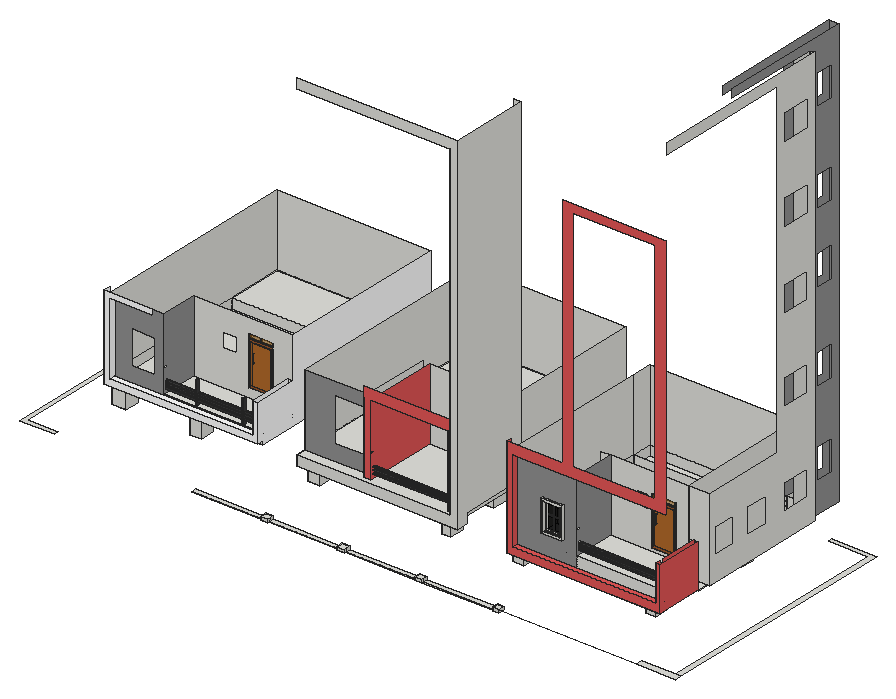
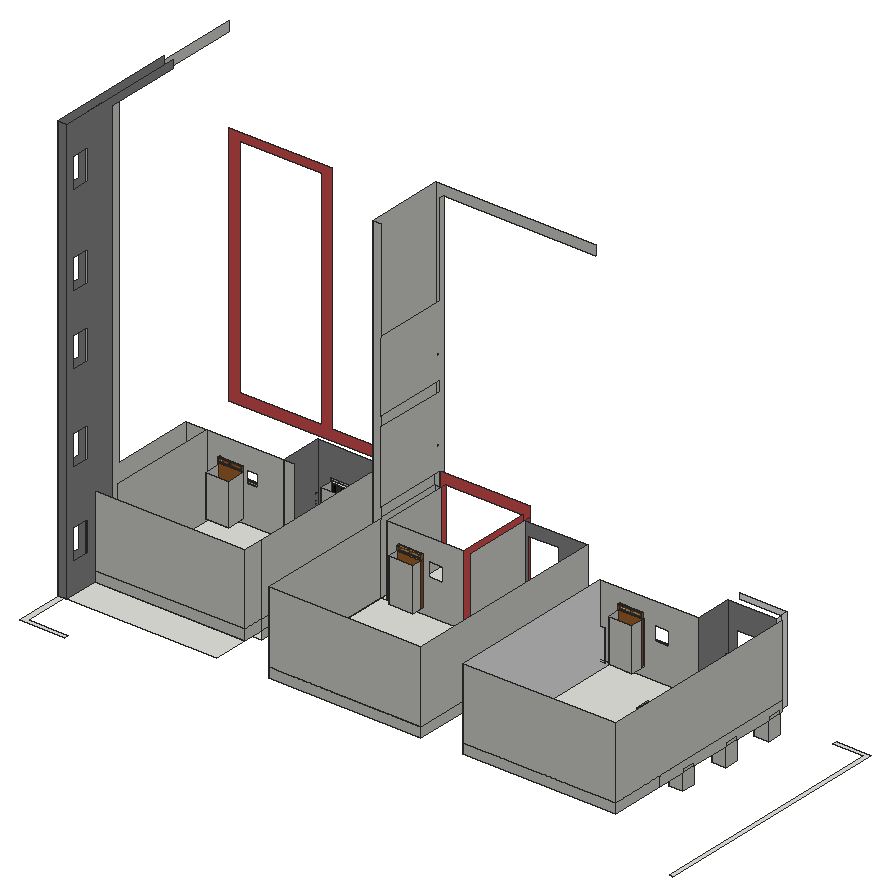
# SketchUp Ruby script. Lengths in inches.
U = 1.inch
M = Sketchup.active_model
def pt(a) = Geom::Point3d.new(a.map { |v| v * U })
def face(e, loops, mat)
  f = e.add_face(loops[0].map { |a| pt(a) })
  loops[1..].each { |l| e.add_face(l.map { |a| pt(a) }).erase! }
  f.material = f.back_material = mat if mat
  f
end
# faces: each face lists its corners as indices into pts; further lists are holes
def faces(e, pts, list, mat = nil) = list.each { |f| face(e, (f[0].is_a?(Array) ? f : [f]).map { |l| l.map { |i| pts[i] } }, mat) }
# xy, xz, yz: faces in a plane at the given z, y or x. An outline is a flat list of corners, or four numbers for a rectangle; further outlines are holes
def ring(l) = l.size == 4 ? [[l[0], l[1]], [l[2], l[1]], [l[2], l[3]], [l[0], l[3]]] : l.each_slice(2).to_a
def flat(e, list, mat, &to3) = list.each { |f| face(e, (f[0].is_a?(Array) ? f : [f]).map { |l| ring(l).map { |u, v| to3.(u, v) } }, mat) }
def xy(e, z, list, mat = nil) = flat(e, list, mat) { |x, y| [x, y, z] }
def xz(e, y, list, mat = nil) = flat(e, list, mat) { |x, z| [x, y, z] }
def yz(e, x, list, mat = nil) = flat(e, list, mat) { |y, z| [x, y, z] }
def lines(e, pts, list) = list.each { |a, b| e.add_line(pt(pts[a]), pt(pts[b])) }
# prism: a flat outline (further loops are holes) pulled along v
def prism(e, loops, v, mat = nil)
  f = face(e, loops, mat); d = Geom::Vector3d.new(v.map { |x| x * U })
  f.pushpull(f.normal.samedirection?(d) ? d.length : -d.length)
end
def box(e, o, s, mat = nil) = prism(e, [[o, [o[0] + s[0], o[1], o[2]], [o[0] + s[0], o[1] + s[1], o[2]], [o[0], o[1] + s[1], o[2]]]], [0, 0, s[2]], mat)
def at(x, y, z, deg = 0) = Geom::Transformation.translation(pt([x, y, z])) * Geom::Transformation.rotation(ORIGIN, Z_AXIS, deg.degrees)
def axes(o, x, y, z) = Geom::Transformation.new([*x, 0, *y, 0, *z, 0, *pt(o).to_a, 1])
def part(name) = M.definitions.add(name)
# library, detail: a bought-in or finely detailed component or shape, given as its bounding box
def library(name, o, s) = part(name).tap { |d| box(d.entities, o, s) }
def detail(e, o, s) = box(e.add_group.entities, o, s)
def put(e, d, t, mat = nil) = e.add_instance(d, t).tap { |i| i.material = mat if mat }
def group(e, t, mat = nil) = e.add_group.tap { |g| g.transformation = t; g.material = mat if mat }.entities
root = M.entities
M.materials.add("Generic").color = [145, 145, 145]
M.materials.add("Generic\#2").color = [229, 87, 87]
M.materials.add("[Color M00]").color = [255, 255, 255]
M.materials.add("[Color M07]").color = [58, 58, 58]
M.materials.add("[Color M08]").color = [45, 45, 45]
M.materials.add("[Translucent Glass Dark Green]").color = [168, 100, 12]
M.materials["[Translucent Glass Dark Green]"].alpha = 0.5
M.materials.add("[Translucent Glass Gray]").color = [0, 0, 0]
M.materials["[Translucent Glass Gray]"].alpha = 0.62
M.materials.add("[Wood Bamboo]").color = [177, 105, 43]
M.materials.add("[Wood Cherry Original]").color = [152, 86, 42]
c1 = part("Group\#10")
xy(c1.entities,0,[[0,1.08,55.8125,6.01]],"[Wood Cherry Original]")
xy(c1.entities,3.96,[[3.96,1.08,51.86,3.01]],"[Wood Bamboo]")
xy(c1.entities,51.66,[[8.63,0,9.88,3.01]],"[Color M08]")
xy(c1.entities,52.54,[[8.63,0.6875,9.88,3.01]],"[Color M08]")
xy(c1.entities,71.82,[[8.63,0.6875,9.88,3.01]],"[Color M08]")
xy(c1.entities,72.69,[[8.63,0,9.88,3.01]],"[Color M08]")
xy(c1.entities,97.36,[[3.96,1.08,51.86,3.01]],"[Wood Bamboo]")
xy(c1.entities,101.3125,[[0,1.08,55.8125,6.01]],"[Wood Bamboo]")
xy(c1.entities,102.55,[[1.23,1.08,27.29,3.01],[27.29,1.08,28.52,1.95],[28.52,1.08,54.58,3.01]],"[Wood Bamboo]")
xy(c1.entities,112.31,[[1.23,1.08,1.23,3.01,27.29,3.01,27.29,1.95,28.52,1.95,28.52,3.01,54.58,3.01,54.58,1.08]],"[Wood Bamboo]")
xy(c1.entities,113.54,[[0,1.08,55.8125,6.01]],"[Wood Bamboo]")
xz(c1.entities,0,[[8.63,51.66,9.88,72.69]],"[Color M08]")
xz(c1.entities,0.6875,[[8.63,52.54,9.88,71.82]])
xz(c1.entities,1.08,[[0,101.3125,55.8125,102.55],[0,102.55,1.23,102.55,1.23,112.31,54.58,112.31,54.58,102.55,55.8125,102.55,55.8125,113.54,0,113.54]],"[Wood Bamboo]")
xz(c1.entities,1.08,[[[0,0,55.8125,101.3125],[3.96,3.96,51.86,97.36]]],"[Wood Cherry Original]")
xz(c1.entities,1.95,[[27.29,102.55,28.52,112.31]],"[Wood Bamboo]")
xz(c1.entities,3.01,[[8.63,71.82,9.88,72.69]])
xz(c1.entities,3.01,[[1.23,102.55,27.29,112.31],[28.52,102.55,54.58,112.31]],"[Translucent Glass Dark Green]")
xz(c1.entities,3.01,[[[3.96,3.96,51.86,97.36],[8.63,71.82,9.88,72.69],[8.63,51.66,9.88,52.54]]],"[Wood Bamboo]")
xz(c1.entities,6.01,[[0,0,55.8125,101.3125],[0,112.31,55.8125,113.54]],"[Wood Bamboo]")
yz(c1.entities,0,[[1.08,101.3125,6.01,113.54]],"[Wood Bamboo]")
yz(c1.entities,0,[[1.08,0,6.01,101.3125]],"[Wood Cherry Original]")
yz(c1.entities,1.23,[[1.08,102.55,3.01,112.31]],"[Wood Bamboo]")
yz(c1.entities,3.96,[[1.08,3.96,3.01,97.36]],"[Wood Bamboo]")
yz(c1.entities,8.63,[[0,51.66,0,72.69,3.01,72.69,3.01,71.82,0.6875,71.82,0.6875,52.54,3.01,52.54,3.01,51.66]],"[Color M08]")
yz(c1.entities,9.88,[[0,51.66,3.01,51.66,3.01,52.54,0.6875,52.54,0.6875,71.82,3.01,71.82,3.01,72.69,0,72.69]],"[Color M08]")
yz(c1.entities,27.29,[[1.95,102.55,3.01,112.31]],"[Wood Bamboo]")
yz(c1.entities,28.52,[[1.95,102.55,3.01,112.31]],"[Wood Bamboo]")
yz(c1.entities,51.86,[[1.08,3.96,3.01,97.36]],"[Wood Bamboo]")
yz(c1.entities,54.58,[[1.08,102.55,3.01,112.31]],"[Wood Bamboo]")
yz(c1.entities,55.8125,[[1.08,101.3125,6.01,113.54]],"[Wood Bamboo]")
yz(c1.entities,55.8125,[[1.08,0,6.01,101.3125]],"[Wood Cherry Original]")
p = [[1.23,3.01,112.31],[1.23,6.01,112.31],[9.24,3.01,71.99],[9.24,0.51,71.99],[9.24,0.51,52.37],[9.24,3.01,52.37]]
lines(c1.entities,p,[[0,1],[2,3],[3,4],[4,5]])
c2 = part("Group\#1")
xy(c2.entities,0,[[0,0,39.9375,6]])
xy(c2.entities,3.79,[[3.79,0,36.15,3]])
xy(c2.entities,60.83,[[3.79,0,36.15,3]])
xy(c2.entities,64.62,[[0,0,39.9375,6]])
xz(c2.entities,0,[[[0,0,39.9375,64.62],[3.79,3.79,36.15,60.83]]])
xz(c2.entities,3,[[18.07,3.79,20.49,3.79,20.49,32.1,36.15,32.1,36.15,34.21,20.49,34.21,20.49,60.83,18.07,60.83,18.07,34.21,3.79,34.21,3.79,32.1,18.07,32.1]],"[Color M08]")
xz(c2.entities,3,[[3.79,3.79,18.07,32.1],[20.49,3.79,36.15,32.1],[3.79,34.21,18.07,60.83],[20.49,34.21,36.15,60.83]],"[Translucent Glass Gray]")
xz(c2.entities,6,[[0,0,39.9375,64.62]],"[Translucent Glass Gray]")
yz(c2.entities,0,[[0,0,6,64.62]])
yz(c2.entities,3.79,[[0,3.79,3,60.83]])
yz(c2.entities,36.15,[[0,3.79,3,60.83]])
yz(c2.entities,39.9375,[[0,0,6,64.62]])
box(root,[317.97,107.54,123.46],[28.18,32.5,52.04])
box(root,[317.97,359.61,128.98],[28.18,32.5,46.52])
box(root,[317.97,233.58,128.98],[28.18,32.5,46.52])
xy(root,77.4375,[[566.41,4.0625,583.85,19.0625],[746.02,4.0625,763.9,19.0625],[927.64,4.0625,943.95,19.0625],[1109.75,4.0625,1124,19.0625],[403.8,5.5,566.41,8.375],
  [583.85,5.5,746.02,8.375],[763.9,5.5,927.64,8.375],[943.95,5.5,1109.75,8.375],[403.8,8.375,566.41,19.0625],[583.85,8.375,746.02,19.0625],
  [763.9,8.375,927.64,19.0625],[943.95,8.375,1109.75,19.0625]])
xy(root,84,[[566.41,4.0625,583.85,19.0625],[746.02,4.0625,763.9,19.0625],[927.64,4.0625,943.95,19.0625],[1109.75,4.0625,1124,19.0625],[1447.36,4.0625,1540.27,19.0625],
  [0,8.375,80.43,8.375,80.43,19.0625,8.1875,19.0625,8.1875,590.625,0,590.625],[1528.71,19.0625,1540.27,19.0625,1540.27,590.625,1435.83,590.625,1435.83,580.6875,1528.71,580.6875]])
xy(root,117.37,[[1385.5,359.61,1409.07,392.11]])
xy(root,123.46,[[135.5,107.54,168.88,107.54,135.5,140.04],[168.88,107.54,168.88,140.04,135.5,140.04],[594.11,107.54,622.68,140.04],[909.52,107.54,930.58,140.04],[1075.83,107.54,1100.54,140.04],
  [1385.5,107.54,1409.07,140.04],[135.5,233.58,168.88,266.08],[1385.5,233.58,1409.07,266.08]])
xy(root,128.98,[[909.52,233.58,930.58,266.08],[135.5,359.61,168.88,392.11],[909.52,359.61,930.58,392.11],[1075.83,359.61,1100.54,392.11]])
xy(root,132.52,[[594.11,359.61,622.68,392.11]])
xy(root,148.75,[[1075.83,88,1435.83,99.8125],[[1075.83,99.8125,1075.83,107.54,1100.54,107.54,1100.54,140.04,1075.83,140.04,1075.83,233.58,1100.54,233.58,1100.54,266.08,1075.83,266.08,1075.83,359.61,1100.54,359.61,1100.54,392.11,1075.83,392.11,1075.83,459.8125,1435.83,459.8125,1435.83,99.8125],[1385.5,359.61,1409.07,392.11],[1385.5,233.58,1409.07,266.08],[1385.5,107.54,1409.07,140.04]],[1075.83,107.54,1100.54,140.04],[1075.83,233.58,1100.54,266.08],[1075.83,359.61,1100.54,392.11]])
xy(root,168,[[[594.11,74.75,594.11,107.54,622.68,107.54,622.68,140.04,594.11,140.04,594.11,233.58,622.68,233.58,622.68,266.08,594.11,266.08,594.11,359.61,622.68,359.61,622.68,392.11,594.11,392.11,594.11,459.8125,954.11,459.8125,954.11,99.8125,972.24,99.8125,972.24,74.75],[909.52,359.61,930.58,392.11],[909.52,233.58,930.58,266.08],[909.52,107.54,930.58,140.04]],[135.5,99.8125,495.5,459.8125],[1413.27,199.25,1435.83,459.8125],[1435.83,199.25,1435.83,459.8125,1451.02,459.8125,1451.02,507.75,1462.21,507.75,1462.21,199.25],[594.11,359.61,622.68,392.11],
  [135.5,459.8125,495.5,590.625],[594.11,459.8125,954.11,590.625],[1075.83,459.8125,1429.21,507.75],[1429.21,459.8125,1435.83,507.75],[1435.83,459.8125,1451.02,507.75],
  [1075.83,507.75,1429.21,590.625],[1429.21,507.75,1435.83,590.625],[1435.83,507.75,1451.02,591.3125],[1429.21,590.625,1435.83,591.3125]])
xy(root,168,[[1091.08,88,1425.14,99.8125]],"Generic\#2")
xy(root,175.5,[[135.5,107.54,168.88,140.04],[135.5,233.58,168.88,266.08],[135.5,359.61,168.88,392.11]])
xy(root,175.5,[[135.5,84.5,495.5,99.8125]],"[Color M00]")
xy(root,189.875,[[147.6875,84.5,482.8125,99.8125]],"[Color M00]")
xy(root,192,[[594.11,74.75,954.11,74.75,954.11,86,940.8,86,940.8,258.8125,758.59,258.8125,758.59,86,741.96,86,741.96,99.8125,594.11,99.8125],[741.96,86,758.59,99.8125],[940.8,86,954.11,99.8125],[[263.03,99.8125,482.8125,187.125],[446.53,103.76,448.09,107.89],[443.78,103.76,445.34,107.89],[336.59,103.76,338.15,107.89],[333.84,103.76,335.4,107.89]],[594.11,99.8125,594.11,459.8125,954.11,459.8125,954.11,258.8125,741.96,258.8125,741.96,99.8125],
  [741.96,99.8125,758.59,258.8125],[940.8,99.8125,954.11,258.8125],[954.11,99.8125,972.24,260.5],[1230.96,99.8125,1425.14,199.25],[333.84,103.76,335.4,107.89],
  [336.59,103.76,338.15,107.89],[443.78,103.76,445.34,107.89],[446.53,103.76,448.09,107.89],[135.5,459.8125,495.5,590.625],[594.11,459.8125,954.11,590.625]])
xy(root,200.58,[[1327.46,199.25,1383.27,240]])
xy(root,201.99,[[263.03,103.34,482.8125,108.98]],"[Color M07]")
xy(root,202.93,[[1230.96,102.74,1425.14,108.3]],"[Color M07]")
xy(root,203.3,[[758.59,90.7,954.11,95.51]],"[Color M07]")
xy(root,205.17,[[758.59,90.7,954.11,95.51]],"[Color M07]")
xy(root,205.37,[[263.03,103.34,482.8125,108.98]],"[Color M07]")
xy(root,205.68,[[1230.96,102.74,1425.14,108.3]],"[Color M07]")
xy(root,205.88,[[856.48,258.8125,912.29,288.3125]])
xy(root,209.56,[[263.03,103.34,482.8125,108.98]],"[Color M07]")
xy(root,209.61,[[1230.96,102.74,1425.14,108.3]],"[Color M07]")
xy(root,210.3,[[758.59,90.7,954.11,95.51]],"[Color M07]")
xy(root,212.17,[[758.59,90.7,954.11,95.51]],"[Color M07]")
xy(root,212.34,[[392.26,187.125,448.07,220.9375]])
xy(root,212.36,[[1230.96,102.74,1425.14,108.3]],"[Color M07]")
xy(root,212.93,[[263.03,103.34,482.8125,108.98]],"[Color M07]")
xy(root,215.76,[[1151.9,93.8125,1200.57,99.8125]])
xy(root,215.99,[[263.03,103.34,482.8125,108.98]],"[Color M07]")
xy(root,216.61,[[1230.96,102.74,1425.14,108.3]],"[Color M07]")
xy(root,217.3,[[758.59,90.7,954.11,95.51]],"[Color M07]")
xy(root,219.17,[[758.59,90.7,954.11,95.51]],"[Color M07]")
xy(root,219.36,[[1230.96,102.74,1425.14,108.3]],"[Color M07]")
xy(root,219.37,[[263.03,103.34,482.8125,108.98]],"[Color M07]")
xy(root,220.13,[[1156.27,93.8125,1196.2,99.8125],[1156.27,99.8125,1196.2,134.3125]])
xz(root,4.0625,[[566.41,77.4375,583.85,84],[746.02,77.4375,763.9,84],[927.64,77.4375,943.95,84],[1109.75,77.4375,1124,84]])
xz(root,19.0625,[[566.41,77.4375,583.85,84],[746.02,77.4375,763.9,84],[927.64,77.4375,943.95,84],[1109.75,77.4375,1124,84]])
xz(root,74.75,[[594.11,168,972.24,168,972.24,983.6875,594.11,983.6875,594.11,960,954.11,960,954.11,192,594.11,192]])
xz(root,84.5,[[135.5,175.5,495.5,175.5,495.5,262.625,482.8125,262.625,482.8125,189.875,147.6875,189.875,147.6875,360,248.28,360,248.28,373.375,135.5,373.375]],"[Color M00]")
xz(root,86,[[741.96,192,758.59,192,758.59,360,940.8,360,940.8,192,954.11,192,954.11,384,741.96,384]],"Generic\#2")
xz(root,88,[[[1075.83,148.75,1435.83,148.75,1435.83,250.36,1425.14,250.36,1425.14,168,1091.08,168,1091.08,360,1448.83,360,1448.83,936,1207.39,936,1207.39,384,1075.83,384],[1230.96,384,1423.39,917.875]]],"Generic\#2")
xz(root,90.7,[[758.59,203.3,954.11,205.17],[758.59,210.3,954.11,212.17],[758.59,217.3,954.11,219.17]],"[Color M07]")
xz(root,93.8125,[[[1151.9,215.76,1200.57,289.12],[1156.27,220.13,1196.2,284.75]]])
xz(root,95.51,[[758.59,203.3,954.11,205.17],[758.59,210.3,954.11,212.17],[758.59,217.3,954.11,219.17]])
xz(root,99.8125,[[135.5,168,495.5,175.5],[954.11,168,972.24,192],[1075.83,168,1091.08,192],[1230.96,168,1425.14,192],[940.8,192,954.11,360],
  [1075.83,192,1091.08,360],[[1151.9,215.76,1200.57,289.12],[1156.27,220.13,1196.2,284.75]]])
xz(root,99.8125,[[[1091.08,168,1230.96,360],[1151.9,215.76,1200.57,289.12]],[[147.6875,189.875,263.03,360],[188.42,224.94,242.3125,304.08]],[[594.11,192,741.96,360],[663.18,229.28,734.35,331.08]]],"Generic")
xz(root,99.8125,[[263.03,189.875,482.8125,192]],"[Color M00]")
xz(root,102.74,[[1230.96,202.93,1425.14,205.68],[1230.96,209.61,1425.14,212.36],[1230.96,216.61,1425.14,219.36]],"[Color M07]")
xz(root,103.34,[[263.03,201.99,482.8125,205.37],[263.03,209.56,482.8125,212.93],[263.03,215.99,482.8125,219.37]],"[Color M07]")
xz(root,103.76,[[333.84,192,335.4,245.62],[336.59,192,338.15,245.93],[443.78,192,445.34,245.06],[446.53,192,448.09,245.06]],"[Color M07]")
xz(root,107.54,[[135.5,123.46,168.88,175.5],[594.11,123.46,622.68,168],[909.52,123.46,930.58,168],[1075.83,123.46,1100.54,148.75],[1385.5,123.46,1409.07,148.75]])
xz(root,107.89,[[333.84,192,335.4,245.62],[336.59,192,338.15,245.93],[443.78,192,445.34,245.06],[446.53,192,448.09,245.06]])
xz(root,108.3,[[1230.96,202.93,1425.14,205.68],[1230.96,209.61,1425.14,212.36],[1230.96,216.61,1425.14,219.36]])
xz(root,108.98,[[263.03,201.99,482.8125,205.37],[263.03,209.56,482.8125,212.93],[263.03,215.99,482.8125,219.37]])
xz(root,134.3125,[[1156.27,220.13,1196.2,284.75]])
xz(root,140.04,[[135.5,123.46,168.88,175.5],[594.11,123.46,622.68,168],[909.52,123.46,930.58,168],[1075.83,123.46,1100.54,148.75],[1385.5,123.46,1409.07,148.75]])
xz(root,187.125,[[[263.03,192,482.8125,192,482.8125,262.625,495.5,262.625,495.5,360,263.03,360],[392.26,212.34,448.07,327.08],[331.98,275.88,365.3125,309.2]]])
xz(root,199.25,[[1413.27,168,1435.83,168,1435.83,250.36,1425.14,250.36,1425.14,192,1413.27,192],[1435.83,168,1462.21,168,1462.21,360,1413.27,360,1413.27,248.125,1425.14,248.125,1425.14,250.36,1435.83,250.36],[1207.39,192,1230.96,360],[[1230.96,192,1413.27,360],[1327.46,200.58,1383.27,314.12],[1292.01,278.6,1317.77,308.93]],[1413.27,192,1425.14,248.125]])
xz(root,220.9375,[[392.26,212.34,448.07,313.66]])
xz(root,233.58,[[1075.83,117.37,1100.54,148.75],[135.5,123.46,168.88,175.5],[1385.5,123.46,1409.07,148.75],[909.52,128.98,930.58,168],[594.11,133.04,622.68,168]])
xz(root,240,[[1327.46,200.58,1383.27,297.87]])
xz(root,258.8125,[[[758.59,192,940.8,360],[856.48,205.88,912.29,321.51],[808.05,275.46,841.375,308.79]]])
xz(root,260.5,[[954.11,192,972.24,983.6875]])
xz(root,266.08,[[135.5,123.46,168.88,175.5],[1385.5,123.46,1409.07,148.75],[909.52,128.98,930.58,168],[1075.83,128.98,1100.54,148.75],[594.11,133.04,622.68,168]])
xz(root,288.3125,[[856.48,205.88,912.29,307.2]])
xz(root,359.61,[[1385.5,117.37,1409.07,148.75],[135.5,128.98,168.88,175.5],[909.52,128.98,930.58,168],[1075.83,128.98,1100.54,148.75],[594.11,132.52,622.68,168]])
xz(root,392.11,[[1385.5,117.37,1409.07,148.75],[135.5,128.98,168.88,175.5],[909.52,128.98,930.58,168],[1075.83,128.98,1100.54,148.75],[594.11,132.52,622.68,168]])
xz(root,459.8125,[[135.5,168,495.5,192],[1075.83,168,1413.27,192],[1413.27,168,1429.21,192],[1429.21,168,1433.58,192],[1433.58,168,1435.83,192],
  [1435.83,168,1451.02,192],[1413.27,192,1429.21,231.86],[1429.21,192,1433.58,231.86],[1433.58,192,1435.83,231.86],[1435.83,192,1451.02,231.86]])
xz(root,507.75,[[1075.83,168,1429.21,192],[1429.21,168,1435.83,192],[1435.83,168,1451.02,192],[1451.02,168,1462.21,1152],[1075.83,192,1429.21,360],
  [1429.21,192,1435.83,360],[1435.83,192,1451.02,360]])
xz(root,590.625,[[135.5,168,495.5,192],[594.11,168,954.11,192],[135.5,192,495.5,360],[594.11,192,954.11,360]])
xz(root,591.3125,[[1429.21,168,1451.02,1170.6875]],"Generic")
yz(root,135.5,[[107.54,123.46,140.04,168],[233.58,123.46,266.08,168],[359.61,128.98,392.11,168],[99.8125,168,99.8125,192,459.8125,192,459.8125,168,392.11,168,392.11,175.5,359.61,175.5,359.61,168,266.08,168,266.08,175.5,233.58,175.5,233.58,168,140.04,168,140.04,175.5,107.54,175.5,107.54,168],[107.54,168,140.04,175.5],
  [233.58,168,266.08,175.5],[359.61,168,392.11,175.5],[459.8125,168,590.625,192],[99.8125,192,590.625,360]])
yz(root,135.5,[[84.5,175.5,99.8125,373.375]],"[Color M00]")
yz(root,147.6875,[[84.5,189.875,99.8125,360]],"[Color M00]")
yz(root,168.88,[[107.54,123.46,140.04,175.5],[233.58,123.46,266.08,175.5],[359.61,128.98,392.11,175.5]])
yz(root,263.03,[[103.34,201.99,108.98,205.37],[103.34,209.56,108.98,212.93],[103.34,215.99,108.98,219.37]])
yz(root,263.03,[[[99.8125,192,106.16,192,106.16,201.99,103.34,201.99,103.34,205.37,108.98,205.37,108.98,201.99,106.16,201.99,106.16,192,187.125,192,187.125,360,99.8125,360],[100.96,245.06,108.98,249.99],[103.34,209.56,108.98,212.93],[103.34,215.99,108.98,219.37],[103.34,222.81,108.98,226.18],[103.34,230.06,108.98,233.43]]],"Generic")
yz(root,333.84,[[103.76,192,107.89,245.62]],"[Color M07]")
yz(root,335.4,[[103.76,192,107.89,245.62]],"[Color M07]")
yz(root,336.59,[[103.76,192,107.89,245.93]],"[Color M07]")
yz(root,338.15,[[103.76,192,107.89,245.93]],"[Color M07]")
yz(root,392.26,[[187.125,212.34,220.9375,313.66]])
yz(root,443.78,[[103.76,192,107.89,245.06]],"[Color M07]")
yz(root,445.34,[[103.76,192,107.89,245.06]],"[Color M07]")
yz(root,446.53,[[103.76,192,107.89,245.06]],"[Color M07]")
yz(root,448.07,[[187.125,212.34,220.9375,313.66]])
yz(root,448.09,[[103.76,192,107.89,245.06]],"[Color M07]")
yz(root,482.8125,[[[84.5,189.875,84.5,262.625,187.125,262.625,187.125,192,99.8125,192,99.8125,189.875],[100.96,245.06,108.98,249.99],[103.34,201.99,108.98,205.37],[103.34,209.56,108.98,212.93],[103.34,215.99,108.98,219.37],[103.34,222.81,108.98,226.18],[103.34,230.06,108.98,233.43]]],"[Color M00]")
yz(root,495.5,[[459.8125,168,590.625,192]])
yz(root,495.5,[[99.8125,168,459.8125,168,459.8125,192,590.625,192,590.625,360,187.125,360,187.125,262.625,84.5,262.625,84.5,175.5,99.8125,175.5]],"[Color M00]")
yz(root,566.41,[[4.0625,77.4375,8.375,84],[8.375,77.4375,19.0625,84]])
yz(root,583.85,[[4.0625,77.4375,8.375,84],[8.375,77.4375,19.0625,84]])
yz(root,594.11,[[107.54,123.46,140.04,168],[359.61,132.52,392.11,168],[233.58,133.04,266.08,168],[74.75,168,459.8125,192],[459.8125,168,590.625,192],
  [99.8125,192,590.625,360]])
yz(root,622.68,[[107.54,123.46,140.04,168],[359.61,132.52,392.11,168]])
yz(root,741.96,[[99.8125,192,258.8125,360]])
yz(root,741.96,[[86,192,99.8125,360]],"Generic\#2")
yz(root,746.02,[[4.0625,77.4375,8.375,84],[8.375,77.4375,19.0625,84]])
yz(root,758.59,[[90.7,203.3,95.51,205.17],[90.7,210.3,95.51,212.17],[90.7,217.3,95.51,219.17]])
yz(root,758.59,[[[86,192,258.8125,360],[87.57,245.73,95.51,251.17],[90.7,203.3,95.51,205.17],[90.7,210.3,95.51,212.17],[90.7,217.3,95.51,219.17],[90.7,224.3,95.51,226.17],[90.7,230.98,95.51,232.86]]],"Generic\#2")
yz(root,763.9,[[4.0625,77.4375,8.375,84],[8.375,77.4375,19.0625,84]])
yz(root,856.48,[[258.8125,205.88,288.3125,307.2]])
yz(root,909.52,[[107.54,123.46,140.04,168],[233.58,128.98,266.08,168],[359.61,128.98,392.11,168]])
yz(root,912.29,[[258.8125,205.88,288.3125,307.2]])
yz(root,927.64,[[4.0625,77.4375,8.375,84],[8.375,77.4375,19.0625,84]])
yz(root,930.58,[[107.54,123.46,140.04,168],[233.58,128.98,266.08,168],[359.61,128.98,392.11,168]])
yz(root,940.8,[[99.8125,192,258.8125,360]])
yz(root,940.8,[[86,192,99.8125,360]],"Generic\#2")
yz(root,943.95,[[4.0625,77.4375,8.375,84],[8.375,77.4375,19.0625,84]])
yz(root,954.11,[[99.8125,168,590.625,192],[[74.75,192,74.75,960,86,960,86,744,258.8125,744,258.8125,576,86,576,86,552,258.8125,552,258.8125,384,86,384,86,192],[87.45,629.96,95.39,635.4],[87.39,437.85,95.33,443.28],[90.58,614.96,95.39,616.83],[90.58,608.08,95.39,609.96],[90.58,601.4,95.39,603.27],[90.58,593.96,95.39,595.83],[90.58,587.21,95.39,589.08],[90.52,395.27,95.33,397.15],[90.27,401.9,95.08,403.77],[90.33,408.77,95.14,410.65],[90.27,416.28,95.08,418.16],[90.39,422.85,95.2,424.72]],[[86,192,99.8125,384],[87.57,245.73,95.51,251.17],[90.7,203.3,95.51,205.17],[90.7,210.3,95.51,212.17],[90.7,217.3,95.51,219.17],[90.7,224.3,95.51,226.17],[90.7,230.98,95.51,232.86]],[99.8125,192,258.8125,360],[258.8125,192,260.5,360],
  [260.5,192,590.625,360]])
yz(root,972.24,[[74.75,168,99.8125,168,99.8125,192,260.5,192,260.5,983.6875,74.75,983.6875]])
yz(root,1075.83,[[233.58,117.37,266.08,148.75],[107.54,123.46,140.04,148.75],[359.61,128.98,392.11,148.75],[99.8125,148.75,459.8125,168],[99.8125,168,459.8125,192],
  [459.8125,168,507.75,192],[99.8125,192,459.8125,360],[459.8125,192,507.75,360]])
yz(root,1075.83,[[88,148.75,99.8125,384]],"Generic\#2")
yz(root,1091.08,[[88,168,99.8125,360]],"Generic\#2")
yz(root,1100.54,[[233.58,117.37,266.08,148.75],[107.54,123.46,140.04,148.75],[359.61,128.98,392.11,148.75]])
yz(root,1109.75,[[4.0625,77.4375,8.375,84],[8.375,77.4375,19.0625,84]])
yz(root,1124,[[4.0625,77.4375,19.0625,84]])
yz(root,1151.9,[[93.8125,215.76,99.8125,289.12]])
yz(root,1156.27,[[93.8125,220.13,99.8125,284.75],[99.8125,220.13,134.3125,284.75]])
yz(root,1196.2,[[93.8125,220.13,99.8125,284.75],[99.8125,220.13,134.3125,284.75]])
yz(root,1200.57,[[93.8125,215.76,99.8125,289.12]])
yz(root,1230.96,[[102.74,202.93,108.3,205.68],[102.74,209.61,108.3,212.36],[102.74,216.61,108.3,219.36]])
yz(root,1230.96,[[[99.8125,192,199.25,360],[100.55,245.43,108.3,250.36],[102.74,202.93,108.3,205.68],[102.74,209.61,108.3,212.36],[102.74,216.61,108.3,219.36],[102.74,223.99,108.3,226.74],[102.74,230.43,108.3,233.18]]],"Generic")
yz(root,1327.46,[[199.25,200.58,240,297.87]])
yz(root,1383.27,[[199.25,200.58,240,297.87]])
yz(root,1385.5,[[359.61,117.37,392.11,148.75],[107.54,123.46,140.04,148.75],[233.58,123.46,266.08,148.75]])
yz(root,1409.07,[[359.61,117.37,392.11,148.75],[107.54,123.46,140.04,148.75],[233.58,123.46,266.08,148.75]])
yz(root,1413.27,[[199.25,168,199.25,360,459.8125,360,459.8125,283.49,421.57,283.49,421.57,231.86,459.8125,231.86,459.8125,168]])
yz(root,1425.14,[[[88,168,99.8125,168,99.8125,192,199.25,192,199.25,250.36,108.3,250.36,108.3,245.43,100.55,245.43,100.55,250.36,88,250.36],[102.74,230.43,108.3,233.18],[102.74,223.99,108.3,226.74],[102.74,216.61,108.3,219.36],[102.74,209.61,108.3,212.36],[102.74,202.93,108.3,205.68]]],"Generic\#2")
yz(root,1429.21,[[[459.8125,168,459.8125,1152,279.74,1152,279.74,1170.6875,591.3125,1170.6875,591.3125,168],[528.77,1023.75,572.96,1095.24],[528.77,809.68,572.96,881.18],[528.77,644.75,572.96,716.24],[528.77,436.87,572.96,508.37],[528.77,239.12,572.96,310.62]]],"Generic")
yz(root,1435.83,[[459.8125,168,507.75,192],[459.8125,192,507.75,192,507.75,360,459.8125,360,459.8125,283.49,481,283.49,481,231.86,459.8125,231.86]])
yz(root,1435.83,[[88,148.75,199.25,250.36]],"Generic\#2")
yz(root,1451.02,[[459.8125,168,507.75,168,507.75,936,507.5625,936,507.5625,1128,507.75,1128,507.75,1152,459.8125,1152]])
yz(root,1451.02,[[[507.75,168,591.3125,168,591.3125,1170.6875,279.74,1170.6875,279.74,1152,507.75,1152],[528.77,1023.75,572.96,1095.24],[528.77,809.68,572.96,881.18],[528.77,644.75,572.96,716.24],[528.77,436.87,572.96,508.37],[528.77,239.12,572.96,310.62]]],"Generic")
yz(root,1462.21,[[[199.25,168,507.75,168,507.75,1152,73.25,1152,73.25,1128,398.12,1128,398.12,360,199.25,360],[416.24,823.79,486.33,886.0625],[416.24,1002.85,486.33,1065.125],[417.16,227.46,485.41,287.89],[417.16,447.34,485.41,507.77],[417.16,642.84,485.41,703.27],[310.17,224.91,363.48,283.71],[215.23,224.34,268.54,283.15]]])
p = [[135.5,99.8125,192],[147.6875,99.8125,192],[482.8125,187.125,192],[495.5,187.125,192],[482.8125,187.125,187.625],[495.5,187.125,187.625],
  [263.03,105.8125,204],[482.8125,105.8125,204],[263.03,105.8125,211],[482.8125,105.8125,211],[263.03,105.8125,218],[482.8125,105.8125,218],
  [1207.39,99.8125,192],[1207.39,199.25,192],[1425.14,99.8125,168],[1435.83,99.8125,168],[482.8125,99.8125,192],[495.5,99.8125,192],
  [1435.83,507.75,192],[1435.83,590.625,192],[758.59,92.91,204],[940.8,92.91,204],[758.59,92.91,211],[940.8,92.91,211],
  [758.59,92.91,218],[940.8,92.91,218],[1230.96,105,204],[1425.14,105,204],[1230.96,105,211],[1425.14,105,211],
  [1230.96,105,218],[1425.14,105,218],[1447.36,4.0625,84],[1124,4.0625,84]]
lines(root,p,[[0,1],[2,3],[4,5],[4,2],[6,7],[8,9],[10,11],[12,13],[14,15],[16,17],[18,19],[20,21],
  [22,23],[24,25],[26,27],[28,29],[30,31],[32,33]])
put(root,c1,at(1327.46,198.17,200.58))
put(root,c1,at(856.48,257.74,205.88))
put(root,c1,at(392.26,187.125,213.54))
put(root,c2,at(1156.27,99.8125,220.13))
